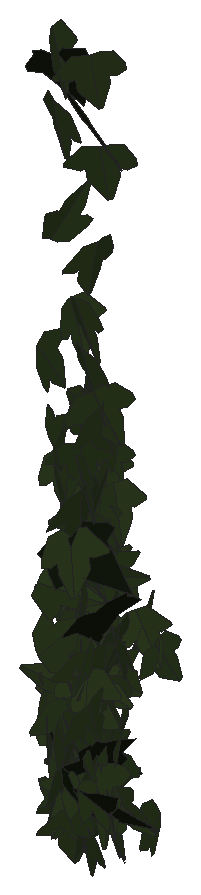
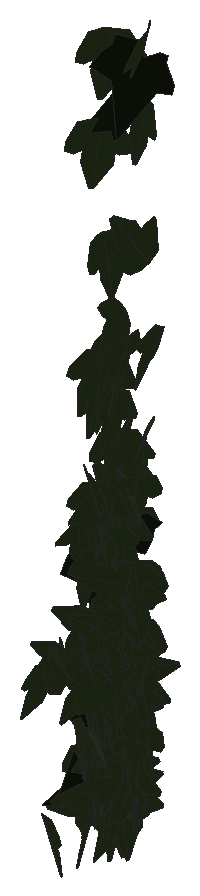
# SketchUp Ruby script. Lengths in inches.
U = 1.inch
M = Sketchup.active_model
def pt(a) = Geom::Point3d.new(a.map { |v| v * U })
def face(e, loops, mat)
  f = e.add_face(loops[0].map { |a| pt(a) })
  loops[1..].each { |l| e.add_face(l.map { |a| pt(a) }).erase! }
  f.material = f.back_material = mat if mat
  f
end
# faces: each face lists its corners as indices into pts; further lists are holes
def faces(e, pts, list, mat = nil) = list.each { |f| face(e, (f[0].is_a?(Array) ? f : [f]).map { |l| l.map { |i| pts[i] } }, mat) }
# xy, xz, yz: faces in a plane at the given z, y or x. An outline is a flat list of corners, or four numbers for a rectangle; further outlines are holes
def ring(l) = l.size == 4 ? [[l[0], l[1]], [l[2], l[1]], [l[2], l[3]], [l[0], l[3]]] : l.each_slice(2).to_a
def flat(e, list, mat, &to3) = list.each { |f| face(e, (f[0].is_a?(Array) ? f : [f]).map { |l| ring(l).map { |u, v| to3.(u, v) } }, mat) }
def xy(e, z, list, mat = nil) = flat(e, list, mat) { |x, y| [x, y, z] }
def xz(e, y, list, mat = nil) = flat(e, list, mat) { |x, z| [x, y, z] }
def yz(e, x, list, mat = nil) = flat(e, list, mat) { |y, z| [x, y, z] }
def lines(e, pts, list) = list.each { |a, b| e.add_line(pt(pts[a]), pt(pts[b])) }
# prism: a flat outline (further loops are holes) pulled along v
def prism(e, loops, v, mat = nil)
  f = face(e, loops, mat); d = Geom::Vector3d.new(v.map { |x| x * U })
  f.pushpull(f.normal.samedirection?(d) ? d.length : -d.length)
end
def box(e, o, s, mat = nil) = prism(e, [[o, [o[0] + s[0], o[1], o[2]], [o[0] + s[0], o[1] + s[1], o[2]], [o[0], o[1] + s[1], o[2]]]], [0, 0, s[2]], mat)
def at(x, y, z, deg = 0) = Geom::Transformation.translation(pt([x, y, z])) * Geom::Transformation.rotation(ORIGIN, Z_AXIS, deg.degrees)
def axes(o, x, y, z) = Geom::Transformation.new([*x, 0, *y, 0, *z, 0, *pt(o).to_a, 1])
def part(name) = M.definitions.add(name)
# library, detail: a bought-in or finely detailed component or shape, given as its bounding box
def library(name, o, s) = part(name).tap { |d| box(d.entities, o, s) }
def detail(e, o, s) = box(e.add_group.entities, o, s)
def put(e, d, t, mat = nil) = e.add_instance(d, t).tap { |i| i.material = mat if mat }
def group(e, t, mat = nil) = e.add_group.tap { |g| g.transformation = t; g.material = mat if mat }.entities
root = M.entities
M.materials.add("efeu1").color = [18, 25, 13]
M.materials.add("efeu2").color = [43, 57, 29]
c1 = part("ivyleaf_10")
p = [[0,0.5,-0.03],[-0.0625,2.02,-0.43],[-0.19,2.01,-0.46],[-0.54,1.05,-0.29],[-0.52,0.625,-0.18],[-0.83,0.76,-0.28],
  [-1.16,0.64,-0.33],[-1.15,0.33,-0.24],[-0.77,-0.39,0.02],[-0.3,-0.51,0.16],[0.04,-0.48,0.23],[-0.02,2.01,-0.4375],
  [-0.06,2.01,-0.43],[0.04,-0.49,0.23],[0.67,-0.49,0.14],[1.38,0.36,-0.2],[1.375,0.51,-0.24],[0.81,0.65,-0.19],
  [0.62,0.59,-0.15],[0.6,1.09,-0.28],[0.5,1.23,-0.31]]
faces(c1.entities,p,[[0,1,2,3,4,5,6,7,8,9,10],[11,12,0,13,14,15,16,17,18,19,20]],"efeu2")
c2 = part("ivyleaf_9")
p = [[1.54,2.16,1.25],[1.36,2.04,1.19],[-0.21,0.99,0.68],[-0.71,1.11,0.82],[-0.85,0.86,0.67],[-0.8,0.17,0.21],
  [-0.9,-0.01,0.1],[-0.67,-0.16,-0.02],[-0.08,-0.08,-0.05],[-0.03,-0.6,-0.4],[0.65,-0.88,-0.66],[0.83,-0.6,-0.49],
  [1.29,-0.42,-0.43],[1.8125,-0.07,-0.26],[1.21,0.44,0.15]]
faces(c2.entities,p,[[0,1,2,3,4,5,6,7,8,9,10,11,12,13,14]],"efeu1")
put(root,c1,axes([509.5,136.41,191.68],[0.41095,0.51714,0.0315],[0.01821,0.0252,-0.66772],[-0.55917,0.38088,0.00141]))
put(root,c1,axes([508.78,136.5,188.49],[0.52609,-0.11777,-0.4389],[0.43666,-0.12229,0.52085],[-0.1823,-0.63279,-0.01898]))
put(root,c1,axes([509.44,136.49,186.62],[-0.58054,0.28027,-0.33803],[0.3012,-0.15358,-0.64462],[-0.31952,-0.65399,0.00652]))
put(root,c1,axes([509.39,136.68,187.47],[0.22135,0.1457,0.60421],[-0.49592,-0.35605,0.26133],[0.41535,-0.50276,-0.00997]))
put(root,c1,axes([508.93,136.17,196.8],[-0.16507,0.50749,0.35914],[-0.12521,0.3256,-0.551],[-0.65101,-0.1913,0.01491]))
put(root,c1,axes([509.74,136.47,192.98],[-0.05253,-0.73593,-0.17359],[-0.00165,0.17412,-0.73768],[0.75613,-0.05074,-0.01367]))
put(root,c1,axes([508.98,136.29,186.54],[-0.21874,0.49829,0.33958],[-0.34367,0.20107,-0.52439],[-0.54393,-0.32743,0.19477]))
put(root,c1,axes([509.15,136.99,184.43],[-0.01177,0.02465,0.61358],[0.06976,-0.58649,0.02672],[0.63391,0.065,0.00846]))
put(root,c1,axes([510.12,136.39,187.26],[-0.07606,-0.67093,-0.29739],[0.0745,0.29038,-0.67417],[0.7301,-0.09953,0.03781]))
put(root,c1,axes([509.33,136.33,186.375],[-0.14703,0.57486,0.22349],[-0.16142,0.18244,-0.60602],[-0.64285,-0.17729,0.10105]))
put(root,c1,axes([509.54,136.86,184.76],[-0.37183,-0.48015,0.37583],[-0.09671,-0.38819,-0.59162],[0.60203,-0.35891,0.13709]))
put(root,c1,axes([509.29,136.58,186.98],[-0.29336,-0.67342,-0.10135],[0.18285,0.02841,-0.71804],[0.656,-0.30907,0.15482]))
put(root,c1,axes([509.74,136.68,188.73],[0.51819,-0.37573,0.01018],[0.00816,-0.00623,-0.63379],[0.40585,0.47987,-0.00026]))
put(root,c2,axes([510.47,136.27,190.16],[0.09935,0.67841,-0.04598],[-0.03115,-0.04068,-0.7116],[-0.73358,0.0936,0.02399]))
put(root,c1,axes([508.61,137.01,187.29],[0.0568,-0.3428,0.51563],[0.2298,-0.45508,-0.35071],[0.60908,0.20367,0.08424]))
put(root,c1,axes([509.01,136.55,205.3],[-0.22138,0.64639,-0.05076],[0.00313,-0.05028,-0.70511],[-0.70008,-0.20462,0.0129]))
put(root,c1,axes([509.61,136.75,193.61],[-0.3784,0.38789,-0.34579],[0.21587,-0.26696,-0.54295],[-0.50778,-0.40255,0.02687]))
put(root,c2,axes([509.41,136.77,184.99],[0.13957,-0.58753,0.29595],[-0.02755,0.28533,0.6247],[-0.70451,-0.12755,0.0342]))
put(root,c1,axes([510.25,136.57,195.81],[-0.44442,-0.48559,-0.25651],[0.24404,0.12905,-0.65632],[0.5352,-0.46208,0.08627]))
put(root,c1,axes([508.87,136.47,190.27],[-0.13917,-0.18146,-0.58168],[0.57186,0.21318,-0.19881],[0.27616,-0.5329,0.11854]))
put(root,c1,axes([509.87,136.17,184.54],[0.16949,0.13451,-0.6664],[0.09206,0.64911,0.16342],[0.70109,-0.11776,0.13965]))
put(root,c1,axes([509.3125,136.45,185.5],[0.10879,-0.59833,-0.40876],[0.00926,0.41446,-0.6042],[0.72457,0.08454,0.0691]))
put(root,c1,axes([509.01,136.59,203.33],[-0.63276,0.27493,0.07282],[-0.0815,0.00384,-0.67243],[-0.29536,-0.59005,0.02955]))
put(root,c1,axes([509.98,136.67,204.96],[-0.48327,-0.4964,-0.09474],[0.08081,0.05515,-0.69479],[0.53905,-0.45331,0.01922]))
put(root,c1,axes([509.72,136.75,187.8125],[0.60471,0.23283,0.02758],[0.02649,0.01009,-0.63066],[-0.25169,0.56046,-0.00011]))
put(root,c1,axes([509.12,136.66,184.46],[0.59381,0.07173,0.20048],[-0.20768,-0.01596,0.57659],[0.07882,-0.58242,0.00889]))
put(root,c1,axes([509.48,136.75,183.98],[-0.35886,-0.62768,-0.01691],[-0.00477,0.0222,-0.72286],[0.62789,-0.35857,-0.01516]))
put(root,c1,axes([510.26,136.64,195.37],[-0.07658,-0.62012,-0.27275],[0.09948,0.25229,-0.64633],[0.72033,-0.10077,0.06026]))
put(root,c2,axes([509.5,136.51,191.7],[0.04548,-0.25662,-0.64608],[0.07733,0.62062,-0.26157],[0.72178,-0.05033,0.06873]))
put(root,c2,axes([509.24,136.82,203.64],[0.59862,-0.37124,0.05877],[0.04047,-0.04556,-0.69358],[0.40354,0.55528,-0.01762]))
put(root,c1,axes([509.25,136.94,183.88],[0.20614,-0.45212,-0.28443],[0.28121,-0.17255,0.48566],[-0.49658,-0.2854,0.15695]))
put(root,c1,axes([509.77,136.86,188.37],[-0.22314,-0.69595,-0.00701],[0.01811,0.00155,-0.73066],[0.69575,-0.22325,0.01677]))
put(root,c1,axes([509.55,136.64,184.28],[-0.41346,0.49571,0.22297],[-0.19754,0.12827,-0.6481],[-0.54882,-0.41961,0.06529]))
put(root,c1,axes([509.59,136.92,186.97],[0.61434,0.20821,-0.04074],[-0.03865,-0.01619,-0.62997],[-0.22553,0.56995,-0.00301]))
put(root,c1,axes([509.78,136.71,183.66],[-0.57895,0.33108,0.19298],[-0.18508,0.07538,-0.65475],[-0.36573,-0.56224,0.02586]))
put(root,c1,axes([510.16,136.84,202.42],[-0.5581,-0.40253,-0.05891],[0.05044,0.03222,-0.68122],[0.43611,-0.51885,0.0034]))
put(root,c2,axes([508.98,136.62,204.79],[0.53742,0.43222,-0.17455],[-0.12211,-0.12565,-0.68516],[-0.48564,0.5099,-0.02087]))
put(root,c1,axes([508.88,136.79,193.29],[-0.27051,0.53644,0.02058],[-0.00691,0.01885,-0.61571],[-0.5797,-0.25054,-0.00226]))
put(root,c1,axes([509.73,137.02,186.11],[0.59465,-0.2442,0.03916],[0.0365,-0.01669,-0.62642],[0.26434,0.55164,-0.00161]))
put(root,c1,axes([509.48,136.9,194.02],[-0.44612,-0.44466,-0.05688],[0.03558,0.04404,-0.63117],[0.48254,-0.41435,-0.00604]))
put(root,c1,axes([509.29,136.54,185.49],[0.24253,-0.02316,0.59797],[-0.37616,0.48583,0.16183],[-0.4947,-0.38077,0.17011]))
put(root,c2,axes([509.65,136.64,184.47],[0.64103,0.07877,0.3011],[0.2952,0.12275,-0.6175],[-0.13365,0.64888,0.08026]))
put(root,c1,axes([508.99,137.03,187.2],[0.57762,0.07277,-0.21816],[-0.2248,-0.02611,-0.56134],[-0.08346,0.5739,0.00213]))
put(root,c1,axes([509.67,136.89,196.55],[-0.57992,0.30426,-0.06336],[0.05166,-0.03913,-0.64177],[-0.33112,-0.53899,0.01083]))
put(root,c1,axes([508.79,136.88,187.99],[-0.46464,0.4774,-0.01559],[0.0099,-0.01192,-0.66836],[-0.51576,-0.43032,0.00122]))
put(root,c1,axes([508.95,136.68,184.8],[0.18435,-0.48745,-0.49833],[-0.09194,0.49396,-0.51719],[0.69101,0.19576,0.06414]))
put(root,c1,axes([509.28,137.03,183.77],[-0.05868,-0.57342,-0.00627],[0.00103,0.00596,-0.59903],[0.61932,-0.05434,0.0004]))
put(root,c1,axes([508.72,136.97,186.32],[0.5283,0.1635,0.31269],[0.30772,0.09599,-0.5364],[-0.20476,0.5661,0.00064]))
put(root,c1,axes([509.82,137.17,185.49],[0.20306,-0.54079,0.12457],[0.04523,-0.11225,-0.59544],[0.5965,0.19261,0.00275]))
put(root,c1,axes([509.61,136.68,190.5625],[0.22367,-0.07943,-0.60008],[-0.35299,0.49103,-0.1923],[0.52065,0.36702,0.12741]))
put(root,c1,axes([508.89,136.57,194.23],[0.15472,0.00837,-0.63128],[-0.11919,0.61364,-0.01829],[0.64469,0.11144,0.14812]))
put(root,c1,axes([509.72,137.08,199.52],[-0.11145,-0.63265,-0.01835],[0.00803,0.01666,-0.66664],[0.68349,-0.10336,0.00484]))
put(root,c1,axes([509.98,136.82,185.04],[0.08181,0.69086,0.22349],[-0.01566,0.22653,-0.69453],[-0.72594,0.07297,0.04017]))
put(root,c2,axes([509.8,136.54,185.73],[0.43523,0.55721,0.27797],[0.17267,0.21784,-0.70704],[-0.59828,0.46823,-0.00184]))
put(root,c1,axes([508.98,137.18,190.03],[-0.41544,-0.43955,0.14295],[-0.09787,-0.10336,-0.60746],[0.48766,-0.39519,-0.00013]))
put(root,c1,axes([509.34,137.07,191.95],[-0.59044,-0.2252,0.01168],[-0.01331,0.00042,-0.61489],[0.24315,-0.54681,-0.00528]))
put(root,c1,axes([508.75,137.16,190.54],[0.17993,0.54607,-0.12316],[-0.05864,-0.10717,-0.59338],[-0.60061,0.17405,0.02104]))
put(root,c1,axes([509.7,137.03,195.52],[-0.4649,0.43601,-0.00196],[0.00129,-0.00146,-0.63722],[-0.4709,-0.43047,0.00018]))
put(root,c1,axes([509.35,137.07,186.27],[0.20181,-0.66324,-0.19052],[0.03127,0.20709,-0.68779],[0.68935,0.18477,0.08697]))
put(root,c1,axes([509.27,137.16,197.68],[-0.52753,0.28683,-0.24215],[0.19649,-0.14918,-0.58806],[-0.34726,-0.52014,0.03512]))
put(root,c1,axes([509.13,136.81,192.73],[0.30354,0.0081,0.5538],[-0.45074,0.37736,0.22312],[-0.35728,-0.4692,0.18901]))
put(root,c1,axes([509.36,137.29,188.86],[0.26048,0.08898,-0.52791],[-0.53337,-0.12022,-0.26596],[-0.15903,0.54898,0.02732]))
put(root,c1,axes([509.02,137.05,184.95],[-0.36012,0.47334,0.20676],[-0.31971,0.01642,-0.55702],[-0.45302,-0.38787,0.22874]))
put(root,c1,axes([509.76,137.35,184.4],[0.52994,-0.19854,0.29205],[0.282,-0.10336,-0.5505],[0.24173,0.55583,0.00195]))
put(root,c1,axes([509.09,137.28,189.05],[-0.35953,0.41198,-0.23714],[0.1209,-0.20199,-0.54954],[-0.49396,-0.3493,0.0381]))
put(root,c1,axes([509.23,137.125,190.39],[0.3741,-0.35905,-0.31304],[-0.20204,0.2372,-0.51817],[0.46392,0.39283,0.02677]))
put(root,c1,axes([509.46,137.62,187.7],[-0.05992,0.16169,-0.5565],[-0.03886,-0.53764,-0.16508],[-0.60246,0.0186,0.06599]))
put(root,c1,axes([509.34,137.29,190.79],[0.42672,-0.43175,-0.10065],[-0.07233,0.0699,-0.60866],[0.47235,0.40074,-0.00227]))
put(root,c1,axes([509.41,137.34,189.64],[0.52592,-0.0246,-0.31934],[-0.33125,0.0147,-0.50708],[0.03094,0.5755,-0.00069]))
put(root,c1,axes([508.64,137.26,193.26],[0.35817,0.48153,0.02651],[0.01504,0.02136,-0.60807],[-0.52056,0.33193,0.00067]))
put(root,c1,axes([509.17,137.47,189],[-0.11169,0.45109,-0.32631],[0.03022,-0.31453,-0.47988],[-0.59267,-0.10105,0.03703]))
put(root,c1,axes([510.32,137.12,186.63],[0.41264,-0.35702,-0.40071],[-0.21349,0.34369,-0.53507],[0.52559,0.4199,0.09726]))
put(root,c1,axes([509.34,137.17,195.31],[-0.0257,-0.55942,-0.25536],[0.15351,0.23391,-0.56858],[0.6417,-0.07836,0.12579]))
put(root,c1,axes([508.63,137.15,199.73],[-0.07172,-0.56595,0.31033],[0.02535,0.29764,0.59253],[-0.69051,0.06971,-0.01048]))
put(root,c1,axes([509.75,137.35,193.125],[0.30293,-0.52415,-0.06711],[-0.03425,0.05622,-0.61826],[0.56933,0.28227,-0.00148]))
put(root,c1,axes([509.02,137.27,185.09],[-0.64546,-0.14454,0.01426],[-0.01446,-0.00297,-0.63947],[0.15614,-0.5978,-0.00027]))
put(root,c1,axes([508.89,137.39,185.6],[0.25618,0.49733,-0.14503],[-0.05433,-0.13048,-0.57294],[-0.55518,0.24225,-0.01086]))
put(root,c1,axes([509.71,137.64,184.18],[0.14649,-0.1933,0.52466],[0.46521,-0.27523,-0.23013],[0.35215,0.44401,0.08576]))
put(root,c1,axes([509.86,137.53,188.3],[-0.02602,-0.55955,0.14825],[-0.01423,-0.1421,-0.58243],[0.62346,-0.0266,-0.00711]))
put(root,c1,axes([509.77,137.42,186.58],[0.46799,-0.35752,-0.13875],[-0.11215,0.08376,-0.58424],[0.39658,0.44559,-0.0015]))
put(root,c1,axes([509.53,137.07,183.8],[0.03104,-0.42127,-0.58695],[-0.02153,0.58669,-0.42222],[0.72216,0.0356,0.01264]))
put(root,c1,axes([508.96,137.375,185.9],[0.13359,0.54164,0.06282],[0.01545,0.05869,-0.57781],[-0.58839,0.12452,-0.00091]))
put(root,c1,axes([509.3,137.41,187.42],[-0.24324,-0.25835,-0.46213],[0.50008,0.10865,-0.30977],[0.24101,-0.48618,0.17635]))
put(root,c1,axes([509.79,137.38,184],[-0.20061,0.2357,-0.52223],[-0.48988,0.24028,0.2918],[0.34485,0.47845,0.11072]))
put(root,c1,axes([509.43,137.42,188.74],[-0.06177,0.01538,0.58788],[-0.58866,0.14981,-0.0616],[-0.16265,-0.54805,-0.00034]))
put(root,c1,axes([509.84,137.57,185.39],[-0.59883,-0.1474,0.07441],[-0.07416,-0.02016,-0.59667],[0.16067,-0.5587,0.0019]))
put(root,c1,axes([509.1875,137.81,189.42],[0.02419,0.46273,-0.31642],[-0.11609,-0.29508,-0.47496],[-0.58673,0.07746,0.08093]))
put(root,c1,axes([509.16,137.62,185.02],[-0.57108,-0.2079,0.02983],[-0.02729,-0.01412,-0.59089],[0.22501,-0.52937,0.00405]))
put(root,c1,axes([509.59,137.7,187.3],[-0.45391,-0.34645,0.10959],[-0.08975,-0.06485,-0.56645],[0.38065,-0.42842,-0.00288]))
put(root,c1,axes([508.75,137.6,197.32],[0.05423,0.60983,0.01305],[0.00235,0.01241,-0.63637],[-0.65875,0.05024,-0.0012]))
put(root,c1,axes([509.45,137.57,189.66],[-0.47412,0.22717,0.30057],[-0.32877,0.0277,-0.50353],[-0.22256,-0.52486,0.10352]))
put(root,c1,axes([510.05,137.55,188.7],[-0.51554,0.3129,0.14474],[-0.12801,0.07304,-0.59358],[-0.347,-0.49183,0.00393]))
put(root,c1,axes([509.16,137.58,191.77],[-0.42286,-0.31714,-0.27859],[0.21699,0.17746,-0.52391],[0.39234,-0.43996,-0.01051]))
put(root,c1,axes([509.92,137.53,183.57],[-0.33736,0.45586,0.19777],[-0.1162,0.1568,-0.57472],[-0.52064,-0.33038,0.00012]))
put(root,c1,axes([509.91,137.7,184.07],[0.20198,-0.04927,0.54797],[0.559,0.13341,-0.17809],[-0.11903,0.54295,0.09348]))
put(root,c1,axes([508.875,137.53,188.58],[0.10818,-0.41533,0.39045],[-0.10705,0.36221,0.44424],[-0.5951,-0.14066,-0.00894]))
put(root,c1,axes([509.07,138.1,185.86],[-0.02703,-0.19677,-0.54798],[0.33356,-0.4456,0.1578],[-0.50767,-0.28231,0.13286]))
put(root,c1,axes([509.86,137.81,188.77],[0.03789,-0.55417,-0.08797],[-0.01117,0.0841,-0.57746],[0.60533,0.03624,-0.00515]))
put(root,c1,axes([508.75,138.05,194.32],[-0.17994,0.44292,0.37975],[0.13957,-0.34151,0.49215],[0.60403,0.21085,-0.00059]))
put(root,c1,axes([509.8,137.39,185.58],[0.07556,-0.03636,-0.61801],[0.02879,0.59792,-0.03478],[0.64233,-0.02252,0.07425]))
put(root,c1,axes([508.97,137.45,185.04],[-0.12162,0.24699,0.5413],[-0.24674,0.4677,-0.28223],[-0.57118,-0.25463,0.00666]))
put(root,c1,axes([508.86,137.98,188.36],[0.33936,0.46884,-0.06753],[-0.03571,-0.05601,-0.58697],[-0.50994,0.31594,-0.00384]))
put(root,c1,axes([509.63,137.57,184.64],[-0.0372,-0.07331,-0.57684],[0.20767,0.5203,-0.08394],[0.56742,-0.19523,-0.0071]))
put(root,c1,axes([509.5625,137.75,187.09],[0.33399,-0.13692,-0.46363],[-0.2768,0.39699,-0.31171],[0.42078,0.36983,0.16295]))
put(root,c1,axes([509.9,137.96,186.22],[0.22296,-0.47726,-0.20446],[-0.08876,0.17865,-0.54078],[0.55034,0.22216,-0.00438]))
put(root,c1,axes([508.68,138.17,191.99],[0.18296,-0.55357,-0.12648],[0.03626,-0.11691,0.60206],[-0.61104,-0.17269,-0.00214]))
put(root,c1,axes([508.83,138.27,192.51],[0.22465,-0.54244,0.0767],[0.03606,-0.06618,-0.60415],[0.59013,0.21054,0.00771]))
put(root,c1,axes([509.25,138.25,193.57],[0.4908,-0.36709,-0.02244],[-0.01813,0.01355,-0.60755],[0.39672,0.45475,-0.00001]))
put(root,c1,axes([509.625,137.83,187.56],[0.10554,0.3687,0.43006],[0.03492,0.4154,-0.39313],[-0.59732,0.08943,0.05301]))
put(root,c1,axes([508.72,138.22,192.21],[0.4386,0.40119,-0.06997],[-0.06023,-0.03926,-0.59358],[-0.43519,0.40977,0.01163]))
put(root,c1,axes([509.52,138.17,192.22],[0.11394,0.58211,-0.01145],[-0.00008,-0.01117,-0.61525],[-0.62879,0.10548,-0.002]))
put(root,c1,axes([509.19,138.21,193.04],[0.0826,0.57419,-0.05355],[-0.07302,-0.04265,-0.59906],[-0.61831,0.08175,0.06359]))
put(root,c1,axes([508.84,138.16,192.75],[-0.17146,0.56954,0.02464],[-0.00642,0.02294,-0.6149],[-0.6156,-0.15887,-0.00045]))
put(root,c1,axes([509.07,138.2,193.24],[-0.45933,-0.36196,-0.17672],[0.17122,0.0751,-0.57905],[0.39646,-0.45179,0.04533]))
put(root,c1,axes([508.75,138.29,190.43],[-0.19263,0.52778,-0.14281],[0.0571,-0.12706,-0.57931],[-0.58621,-0.1858,-0.0095]))
put(root,c1,axes([510.5,138.38,183.52],[0.40747,-0.36789,-0.23715],[-0.16253,0.17212,-0.54777],[0.43829,0.40585,0.01734]))
put(root,c1,axes([508.6,138.13,190.9375],[0.02353,-0.27012,0.54425],[0.05213,0.52273,0.27852],[-0.63389,0.03296,0.04311]))
put(root,c1,axes([509.16,138.65,189.33],[0.29785,-0.48416,0.01343],[0.01073,-0.00921,-0.57947],[0.52297,0.27594,0.00423]))
put(root,c1,axes([508.91,138.47,189.61],[-0.15967,-0.14617,0.55008],[0.52309,0.22275,0.20481],[-0.2786,0.502,0.06929]))
put(root,c1,axes([509.15,138.37,191.43],[0.00424,0.52846,0.22024],[-0.14268,0.20684,-0.53426],[-0.59808,-0.0456,0.12902]))
put(root,c1,axes([508.7,138.29,189.6],[0.19083,0.22618,-0.51322],[0.33056,0.3871,0.2985],[0.4842,-0.35341,-0.00151]))
put(root,c1,axes([508.65,138.68,188.26],[-0.50271,0.05219,-0.30738],[0.30751,-0.09564,-0.48393],[-0.10248,-0.54302,0.05569]))
put(root,c1,axes([509.83,138.65,188.63],[0.48227,0.17687,0.30113],[0.27734,0.13664,-0.49867],[-0.23951,0.51437,0.02893]))
put(root,c1,axes([509.85,138.65,188.21],[0.24233,-0.41418,0.3092],[-0.16203,0.2568,0.48982],[-0.52624,-0.26979,-0.00843]))
put(root,c1,axes([509.16,138.54,189.84],[0.02252,0.44511,0.35077],[-0.03602,0.33791,-0.46163],[-0.60206,-0.00357,0.04074]))
put(root,c1,axes([510.34,138.79,187.99],[-0.09294,-0.47616,-0.28204],[0.21358,0.22903,-0.48348],[0.55193,-0.16881,0.1396]))
